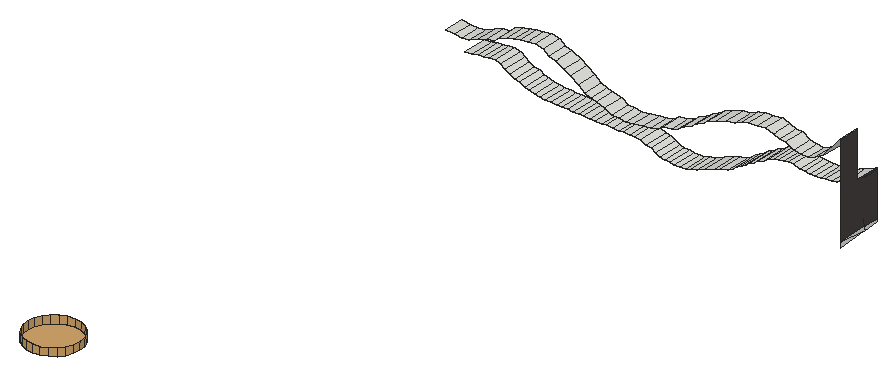
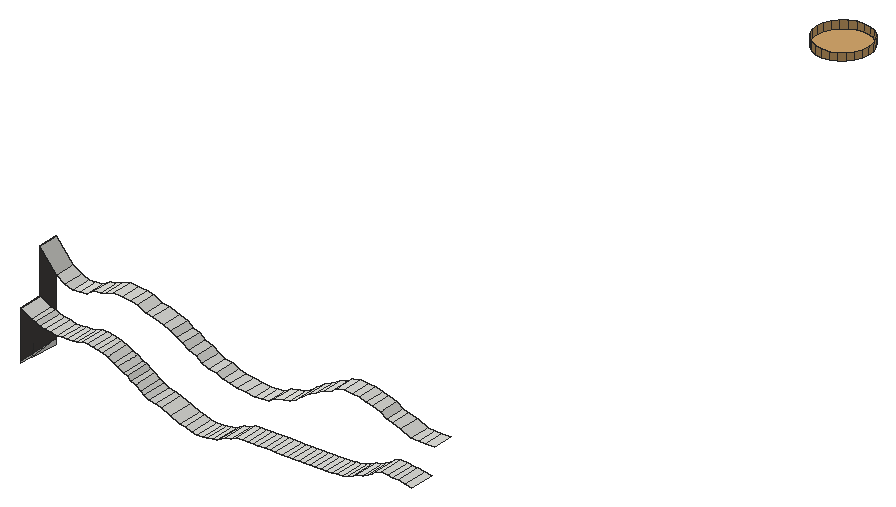
# SketchUp Ruby script. Lengths in inches.
U = 1.inch
M = Sketchup.active_model
def pt(a) = Geom::Point3d.new(a.map { |v| v * U })
def face(e, loops, mat)
  f = e.add_face(loops[0].map { |a| pt(a) })
  loops[1..].each { |l| e.add_face(l.map { |a| pt(a) }).erase! }
  f.material = f.back_material = mat if mat
  f
end
# faces: each face lists its corners as indices into pts; further lists are holes
def faces(e, pts, list, mat = nil) = list.each { |f| face(e, (f[0].is_a?(Array) ? f : [f]).map { |l| l.map { |i| pts[i] } }, mat) }
# xy, xz, yz: faces in a plane at the given z, y or x. An outline is a flat list of corners, or four numbers for a rectangle; further outlines are holes
def ring(l) = l.size == 4 ? [[l[0], l[1]], [l[2], l[1]], [l[2], l[3]], [l[0], l[3]]] : l.each_slice(2).to_a
def flat(e, list, mat, &to3) = list.each { |f| face(e, (f[0].is_a?(Array) ? f : [f]).map { |l| ring(l).map { |u, v| to3.(u, v) } }, mat) }
def xy(e, z, list, mat = nil) = flat(e, list, mat) { |x, y| [x, y, z] }
def xz(e, y, list, mat = nil) = flat(e, list, mat) { |x, z| [x, y, z] }
def yz(e, x, list, mat = nil) = flat(e, list, mat) { |y, z| [x, y, z] }
def lines(e, pts, list) = list.each { |a, b| e.add_line(pt(pts[a]), pt(pts[b])) }
# prism: a flat outline (further loops are holes) pulled along v
def prism(e, loops, v, mat = nil)
  f = face(e, loops, mat); d = Geom::Vector3d.new(v.map { |x| x * U })
  f.pushpull(f.normal.samedirection?(d) ? d.length : -d.length)
end
def box(e, o, s, mat = nil) = prism(e, [[o, [o[0] + s[0], o[1], o[2]], [o[0] + s[0], o[1] + s[1], o[2]], [o[0], o[1] + s[1], o[2]]]], [0, 0, s[2]], mat)
def at(x, y, z, deg = 0) = Geom::Transformation.translation(pt([x, y, z])) * Geom::Transformation.rotation(ORIGIN, Z_AXIS, deg.degrees)
def axes(o, x, y, z) = Geom::Transformation.new([*x, 0, *y, 0, *z, 0, *pt(o).to_a, 1])
def part(name) = M.definitions.add(name)
# library, detail: a bought-in or finely detailed component or shape, given as its bounding box
def library(name, o, s) = part(name).tap { |d| box(d.entities, o, s) }
def detail(e, o, s) = box(e.add_group.entities, o, s)
def put(e, d, t, mat = nil) = e.add_instance(d, t).tap { |i| i.material = mat if mat }
def group(e, t, mat = nil) = e.add_group.tap { |g| g.transformation = t; g.material = mat if mat }.entities
root = M.entities
M.materials.add("[Field Square Tile]").color = [211, 167, 108]
M.materials.add("[Granite Tile]1").color = [68, 65, 63]
xy(root,250.6875,[[3013.293,492.582,3012.581,492.675,3011.918,492.95,3011.348,493.387,3010.911,493.957,3010.636,494.62,3010.543,495.332,3010.636,496.043,3010.911,496.707,3011.348,497.276,3011.918,497.713,3012.581,497.988,3013.293,498.082,3014.004,497.988,3014.668,497.713,3015.237,497.276,3015.674,496.707,3015.949,496.043,3016.043,495.332,3015.949,494.62,3015.674,493.957,3015.237,493.387,3014.668,492.95,3014.004,492.675]],"[Field Square Tile]")
yz(root,3043.095,[[561.053,240.932,561.053,241.519,564.151,241.17],[564.185,241.167,564.151,241.17,564.184,241.173],[564.151,241.17,561.053,241.519,564.144,241.519,564.184,241.173],[564.184,241.173,564.144,241.519,565.74,241.519,565.74,241.293]])
yz(root,3043.095,[[561.053,241.519,561.053,251.165,563.178,251.165,563.178,246.426,565.74,246.426,565.74,241.519]],"[Granite Tile]1")
p = [[3023.517,563.178,241.17],[3023.517,565.74,241.17],[3023.987,565.74,241.121],[3023.987,563.178,241.121],[3024.593,565.74,241.09],[3024.593,563.178,241.09],
  [3025.16,565.74,241.138],[3025.16,563.178,241.138],[3025.8,565.74,241.346],[3025.8,563.178,241.346],[3022.519,563.178,241.332],[3022.519,565.74,241.332],
  [3022.987,565.74,241.243],[3022.987,563.178,241.243],[3022.1,563.178,241.566],[3022.1,565.74,241.566],[3026.391,565.74,241.456],[3026.391,563.178,241.456],
  [3027.326,565.74,241.847],[3027.326,563.178,241.847],[3021.594,563.178,241.837],[3021.594,565.74,241.837],[3021.021,563.178,241.967],[3021.021,565.74,241.967],
  [3028.331,565.74,242.229],[3028.331,563.178,242.229],[3020.44,563.178,242.199],[3020.44,565.74,242.199],[3019.814,563.178,242.277],[3019.814,565.74,242.277],
  [3028.892,565.74,242.424],[3028.892,563.178,242.424],[3013.967,563.178,242.35],[3013.967,565.74,242.35],[3014.549,565.74,242.342],[3014.549,563.178,242.342],
  [3015.131,565.74,242.334],[3015.131,563.178,242.334],[3015.713,565.74,242.326],[3015.713,563.178,242.326],[3016.433,565.74,242.317],[3016.433,563.178,242.317],
  [3016.903,565.74,242.312],[3016.903,563.178,242.312],[3017.544,565.74,242.304],[3017.544,563.178,242.304],[3018.208,565.74,242.296],[3018.208,563.178,242.296],
  [3018.66,565.74,242.291],[3018.66,563.178,242.291],[3019.298,565.74,242.283],[3019.298,563.178,242.283],[3010.485,563.178,242.466],[3010.485,565.74,242.466],
  [3011.061,565.74,242.428],[3011.061,563.178,242.428],[3011.64,565.74,242.403],[3011.64,563.178,242.403],[3012.22,565.74,242.385],[3012.22,563.178,242.385],
  [3012.802,565.74,242.371],[3012.802,563.178,242.371],[3013.384,565.74,242.36],[3013.384,563.178,242.36],[3029.61,565.74,242.605],[3029.61,563.178,242.605],
  [3009.357,563.178,242.599],[3009.357,565.74,242.599],[3009.917,565.74,242.518],[3009.917,563.178,242.518],[3008.804,563.178,242.75],[3008.804,565.74,242.75],
  [3030.123,565.74,242.907],[3030.123,563.178,242.907],[3008.316,563.178,242.921],[3008.316,565.74,242.921],[3007.825,563.178,243.216],[3007.825,565.74,243.216],
  [3030.495,565.74,243.144],[3030.495,563.178,243.144],[3031.044,565.74,243.516],[3031.044,563.178,243.516],[3007.277,563.178,243.332],[3007.277,565.74,243.332],
  [3006.732,563.178,243.589],[3006.732,565.74,243.589],[3031.518,565.74,243.711],[3031.518,563.178,243.711],[3006.251,563.178,243.88],[3006.251,565.74,243.88],
  [3031.849,565.74,244.02],[3031.849,563.178,244.02],[3005.874,563.178,244.194],[3005.874,565.74,244.194],[3002.086,563.178,243.992],[3002.086,565.74,243.992],
  [3002.789,565.74,244.076],[3002.789,563.178,244.076],[3032.293,565.74,244.206],[3032.293,563.178,244.206],[3003.488,565.74,244.207],[3003.488,563.178,244.207],
  [3004.073,565.74,244.266],[3004.073,563.178,244.266],[3005.277,563.178,244.387],[3005.277,565.74,244.387],[3032.882,565.74,244.569],[3032.882,563.178,244.569],
  [3004.614,565.74,244.296],[3004.614,563.178,244.296],[3033.352,565.74,244.757],[3033.352,563.178,244.757],[3033.969,565.74,245.125],[3033.969,563.178,245.125],
  [3019.165,561.053,245.064],[3019.165,563.178,245.064],[3019.875,563.178,244.949],[3019.875,561.053,244.949],[3020.589,563.178,244.867],[3020.589,561.053,244.867],
  [3021.495,563.178,245.007],[3021.495,561.053,245.007],[3022.439,563.178,245.121],[3022.439,561.053,245.121],[3018.452,561.053,245.459],[3018.452,563.178,245.459],
  [3023.204,563.178,245.254],[3023.204,561.053,245.254],[3034.473,565.74,245.32],[3034.473,563.178,245.32],[3038.174,563.178,245.272],[3038.174,565.74,245.272],
  [3038.732,565.74,245.235],[3038.732,563.178,245.235],[3039.286,565.74,245.216],[3039.286,563.178,245.216],[3039.851,565.74,245.34],[3039.851,563.178,245.34],
  [3023.956,563.178,245.41],[3023.956,561.053,245.41],[3034.955,565.74,245.411],[3034.955,563.178,245.411],[3036.521,563.178,245.552],[3036.521,565.74,245.552],
  [3037.129,565.74,245.346],[3037.129,563.178,245.346],[3037.623,565.74,245.309],[3037.623,563.178,245.309],[3040.483,565.74,245.423],[3040.483,563.178,245.423],
  [3024.59,563.178,245.775],[3024.59,561.053,245.775],[3035.503,565.74,245.481],[3035.503,563.178,245.481],[3041.061,565.74,245.516],[3041.061,563.178,245.516],
  [3017.577,561.053,245.671],[3017.577,563.178,245.671],[3035.985,565.74,245.59],[3035.985,563.178,245.59],[3041.441,565.74,245.763],[3041.441,563.178,245.763],
  [3016.902,561.053,245.834],[3016.902,563.178,245.834],[3016.314,561.053,246.129],[3016.314,563.178,246.129],[3025.386,563.178,245.88],[3025.386,561.053,245.88],
  [3041.91,565.74,245.896],[3041.91,563.178,245.896],[3026.099,563.178,246.16],[3026.099,561.053,246.16],[3043.095,565.74,246.426],[3043.095,563.178,246.426],
  [3015.683,561.053,246.633],[3015.683,563.178,246.633],[3026.696,563.178,246.573],[3026.696,561.053,246.573],[3014.869,561.053,247.185],[3014.869,563.178,247.185],
  [3027.486,563.178,246.902],[3027.486,561.053,246.902],[3002.692,561.053,246.79],[3002.692,563.178,246.79],[3003.471,563.178,246.747],[3003.471,561.053,246.747],
  [3004.218,563.178,246.831],[3004.218,561.053,246.831],[3001.738,561.053,246.838],[3001.738,563.178,246.838],[3005.26,563.178,247.251],[3005.26,561.053,247.251],
  [3028.088,563.178,247.347],[3028.088,561.053,247.347],[3014.157,561.053,247.553],[3014.157,563.178,247.553],[3006.134,563.178,247.546],[3006.134,561.053,247.546],
  [3028.762,563.178,247.615],[3028.762,561.053,247.615],[3006.796,563.178,247.657],[3006.796,561.053,247.657],[3013.266,561.053,248.059],[3013.266,563.178,248.059],
  [3029.349,563.178,248.057],[3029.349,561.053,248.057],[3007.429,563.178,248.162],[3007.429,561.053,248.162],[3012.575,561.053,248.257],[3012.575,563.178,248.257],
  [3030.114,563.178,248.322],[3030.114,561.053,248.322],[3008.223,563.178,248.408],[3008.223,561.053,248.408],[3038.911,561.053,248.295],[3038.911,563.178,248.295],
  [3039.62,563.178,248.218],[3039.62,561.053,248.218],[3040.437,563.178,248.558],[3040.437,561.053,248.558],[3012.044,561.053,248.687],[3012.044,563.178,248.687],
  [3031.225,563.178,248.655],[3031.225,561.053,248.655],[3038.2,561.053,248.42],[3038.2,563.178,248.42],[3008.922,563.178,248.521],[3008.922,561.053,248.521],
  [3037.403,561.053,248.895],[3037.403,563.178,248.895],[3009.616,563.178,248.723],[3009.616,561.053,248.723],[3041.372,563.178,249.022],[3041.372,561.053,249.022],
  [3010.315,563.178,248.801],[3010.315,561.053,248.801],[3011.212,561.053,248.851],[3011.212,563.178,248.851],[3031.998,563.178,248.795],[3031.998,561.053,248.795],
  [3032.861,563.178,249.194],[3032.861,561.053,249.194],[3036.699,561.053,248.962],[3036.699,563.178,248.962],[3036.06,561.053,249.206],[3036.06,563.178,249.206],
  [3043.095,563.178,251.165],[3043.095,561.053,251.165],[3033.534,563.178,249.323],[3033.534,561.053,249.323],[3035.315,561.053,249.478],[3035.315,563.178,249.478],
  [3034.457,563.178,249.406],[3034.457,561.053,249.406],[3013.293,492.582,251.5],[3012.581,492.675,251.5],[3012.581,492.675,250.6875],[3013.293,492.582,250.6875],
  [3014.004,492.675,251.5],[3014.004,492.675,250.6875],[3011.918,492.95,251.5],[3011.918,492.95,250.6875],[3014.668,492.95,251.5],[3014.668,492.95,250.6875],
  [3011.348,493.387,251.5],[3011.348,493.387,250.6875],[3015.237,493.387,251.5],[3015.237,493.387,250.6875],[3010.911,493.957,251.5],[3010.911,493.957,250.6875],
  [3015.674,493.957,251.5],[3015.674,493.957,250.6875],[3010.636,494.62,251.5],[3010.636,494.62,250.6875],[3015.949,494.62,251.5],[3015.949,494.62,250.6875],
  [3010.543,495.332,251.5],[3010.543,495.332,250.6875],[3016.043,495.332,251.5],[3016.043,495.332,250.6875],[3010.636,496.043,251.5],[3010.636,496.043,250.6875],
  [3015.949,496.043,251.5],[3015.949,496.043,250.6875],[3010.911,496.707,251.5],[3010.911,496.707,250.6875],[3015.674,496.707,251.5],[3015.674,496.707,250.6875],
  [3011.348,497.276,251.5],[3011.348,497.276,250.6875],[3015.237,497.276,251.5],[3015.237,497.276,250.6875],[3011.918,497.713,251.5],[3011.918,497.713,250.6875],
  [3014.668,497.713,251.5],[3014.668,497.713,250.6875],[3012.581,497.988,251.5],[3012.581,497.988,250.6875],[3014.004,497.988,251.5],[3014.004,497.988,250.6875],
  [3013.293,498.082,251.5],[3013.293,498.082,250.6875],[3043.095,564.963,246.171],[3043.095,563.948,246.265],[3043.095,565.74,246.273],[3043.095,564.144,241.519],
  [3043.095,564.042,242.384]]
faces(root,p,[[0,1,2,3],[3,2,4,5],[5,4,6,7],[7,6,8,9],[10,11,12,13],[13,12,1,0],[14,15,11,10],[9,8,16,17],
  [17,16,18,19],[20,21,15,14],[22,23,21,20],[19,18,24,25],[26,27,23,22],[28,29,27,26],[25,24,30,31],[32,33,34,35],
  [35,34,36,37],[37,36,38,39],[39,38,40,41],[41,40,42,43],[43,42,44,45],[45,44,46,47],[47,46,48,49],[49,48,50,51],
  [51,50,29,28],[52,53,54,55],[55,54,56,57],[57,56,58,59],[59,58,60,61],[61,60,62,63],[63,62,33,32],[31,30,64,65],
  [66,67,68,69],[69,68,53,52],[70,71,67,66],[65,64,72,73],[74,75,71,70],[76,77,75,74],[73,72,78,79],[79,78,80,81],
  [82,83,77,76],[84,85,83,82],[81,80,86,87],[88,89,85,84],[87,86,90,91],[92,93,89,88],[94,95,96,97],[91,90,98,99],
  [97,96,100,101],[101,100,102,103],[104,105,93,92],[99,98,106,107],[103,102,108,109],[109,108,105,104],[107,106,110,111],[111,110,112,113],
  [114,115,116,117],[117,116,118,119],[119,118,120,121],[121,120,122,123],[124,125,115,114],[123,122,126,127],[113,112,128,129],[130,131,132,133],
  [133,132,134,135],[135,134,136,137],[127,126,138,139],[129,128,140,141],[142,143,144,145],[145,144,146,147],[147,146,131,130],[137,136,148,149],
  [139,138,150,151],[141,140,152,153],[149,148,154,155],[156,157,125,124],[153,152,158,159],[155,154,160,161],[159,158,143,142],[162,163,157,156],
  [164,165,163,162],[151,150,166,167],[161,160,168,169],[167,166,170,171],[169,168,172,173],[174,175,165,164],[171,170,176,177],[178,179,175,174],
  [177,176,180,181],[182,183,184,185],[185,184,186,187],[188,189,183,182],[187,186,190,191],[181,180,192,193],[194,195,179,178],[191,190,196,197],
  [193,192,198,199],[197,196,200,201],[202,203,195,194],[199,198,204,205],[201,200,206,207],[208,209,203,202],[205,204,210,211],[207,206,212,213],
  [214,215,216,217],[217,216,218,219],[220,221,209,208],[211,210,222,223],[224,225,215,214],[213,212,226,227],[228,229,225,224],[227,226,230,231],
  [219,218,232,233],[231,230,234,235],[236,237,221,220],[223,222,238,239],[235,234,237,236],[239,238,240,241],[242,243,229,228],[244,245,243,242],
  [233,232,246,247],[241,240,248,249],[250,251,245,244],[249,248,252,253],[253,252,251,250]])
faces(root,p,[[254,255,256,257],[258,254,257,259],[255,260,261,256],[262,258,259,263],[260,264,265,261],[266,262,263,267],[264,268,269,265],[270,266,267,271],
  [268,272,273,269],[274,270,271,275],[272,276,277,273],[278,274,275,279],[276,280,281,277],[282,278,279,283],[280,284,285,281],[286,282,283,287],
  [284,288,289,285],[290,286,287,291],[288,292,293,289],[294,290,291,295],[292,296,297,293],[298,294,295,299],[296,300,301,297],[300,298,299,301]],"[Field Square Tile]")
lines(root,p,[[302,303],[304,302],[305,306]])
